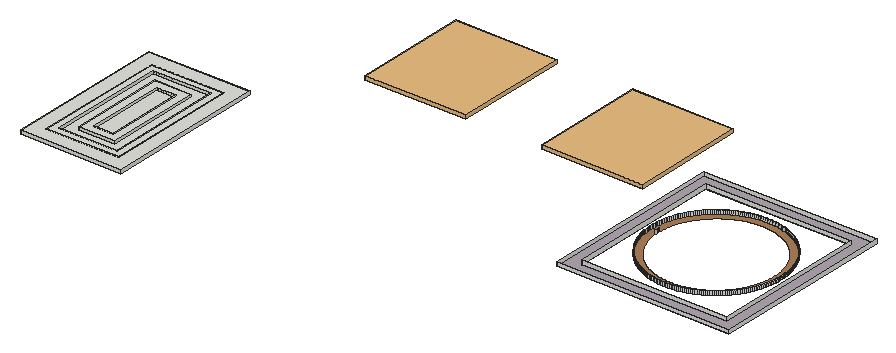
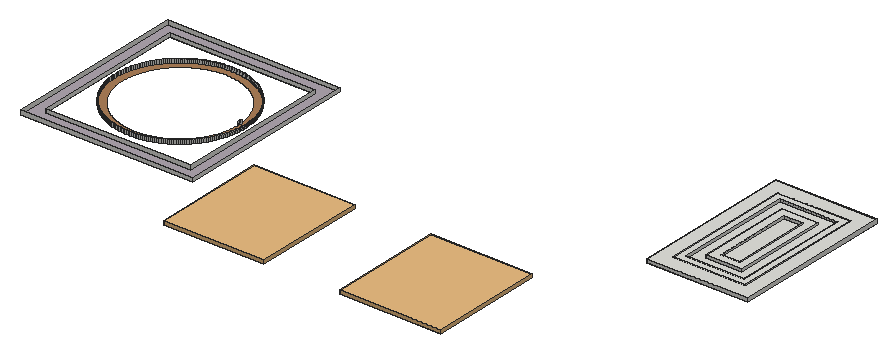
# SketchUp Ruby script. Lengths in inches.
U = 1.inch
M = Sketchup.active_model
def pt(a) = Geom::Point3d.new(a.map { |v| v * U })
def face(e, loops, mat)
  f = e.add_face(loops[0].map { |a| pt(a) })
  loops[1..].each { |l| e.add_face(l.map { |a| pt(a) }).erase! }
  f.material = f.back_material = mat if mat
  f
end
# faces: each face lists its corners as indices into pts; further lists are holes
def faces(e, pts, list, mat = nil) = list.each { |f| face(e, (f[0].is_a?(Array) ? f : [f]).map { |l| l.map { |i| pts[i] } }, mat) }
# xy, xz, yz: faces in a plane at the given z, y or x. An outline is a flat list of corners, or four numbers for a rectangle; further outlines are holes
def ring(l) = l.size == 4 ? [[l[0], l[1]], [l[2], l[1]], [l[2], l[3]], [l[0], l[3]]] : l.each_slice(2).to_a
def flat(e, list, mat, &to3) = list.each { |f| face(e, (f[0].is_a?(Array) ? f : [f]).map { |l| ring(l).map { |u, v| to3.(u, v) } }, mat) }
def xy(e, z, list, mat = nil) = flat(e, list, mat) { |x, y| [x, y, z] }
def xz(e, y, list, mat = nil) = flat(e, list, mat) { |x, z| [x, y, z] }
def yz(e, x, list, mat = nil) = flat(e, list, mat) { |y, z| [x, y, z] }
def lines(e, pts, list) = list.each { |a, b| e.add_line(pt(pts[a]), pt(pts[b])) }
# prism: a flat outline (further loops are holes) pulled along v
def prism(e, loops, v, mat = nil)
  f = face(e, loops, mat); d = Geom::Vector3d.new(v.map { |x| x * U })
  f.pushpull(f.normal.samedirection?(d) ? d.length : -d.length)
end
def box(e, o, s, mat = nil) = prism(e, [[o, [o[0] + s[0], o[1], o[2]], [o[0] + s[0], o[1] + s[1], o[2]], [o[0], o[1] + s[1], o[2]]]], [0, 0, s[2]], mat)
def at(x, y, z, deg = 0) = Geom::Transformation.translation(pt([x, y, z])) * Geom::Transformation.rotation(ORIGIN, Z_AXIS, deg.degrees)
def axes(o, x, y, z) = Geom::Transformation.new([*x, 0, *y, 0, *z, 0, *pt(o).to_a, 1])
def part(name) = M.definitions.add(name)
# library, detail: a bought-in or finely detailed component or shape, given as its bounding box
def library(name, o, s) = part(name).tap { |d| box(d.entities, o, s) }
def detail(e, o, s) = box(e.add_group.entities, o, s)
def put(e, d, t, mat = nil) = e.add_instance(d, t).tap { |i| i.material = mat if mat }
def group(e, t, mat = nil) = e.add_group.tap { |g| g.transformation = t; g.material = mat if mat }.entities
root = M.entities
M.materials.add("01 - Default1").color = [173, 128, 89]
M.materials.add("[0124_Purple]").color = [175, 166, 175]
c1 = library("Group\#54",[0,0,-6],[168,189,6])
c2 = library("Group\#57",[0,0,-6],[168,189,6])
xy(root,111,[[[761.98,172.26,1049.98,478.26],[785.98,196.26,1025.98,454.26]]],"[0124_Purple]")
xy(root,111.3125,[[[905.89,217.26,903.06,217.3,900.23,217.41,897.41,217.6,894.6,217.86,891.79,218.19,888.99,218.6,886.21,219.08,883.43,219.64,880.68,220.26,877.9375,220.96,875.22,221.73,872.52,222.57,869.84,223.48,867.1875,224.46,864.5625,225.51,861.97,226.63,859.4,227.82,856.86,229.07,854.36,230.39,851.9,231.77,849.47,233.22,847.08,234.73,844.73,236.3,842.42,237.9375,840.16,239.63,837.94,241.38,835.77,243.19,833.64,245.06,831.57,246.98,829.55,248.95,827.57,250.98,825.66,253.06,823.79,255.1875,821.99,257.36,820.24,259.58,818.55,261.85,816.92,264.16,815.35,266.51,813.84,268.91,812.4,271.34,811.02,273.81,809.71,276.31,808.46,278.85,807.28,281.41,806.16,284.01,805.12,286.64,804.14,289.29,803.24,291.97,802.4,294.67,801.63,297.39,800.94,300.13,800.32,302.89,799.77,305.67,799.29,308.45,798.89,311.25,798.5625,314.06,798.3,316.875,798.12,319.7,798.01,322.52,797.98,325.35,798.02,328.18,798.13,331,798.32,333.82,798.58,336.64,798.91,339.45,799.32,342.24,799.8,345.03,800.36,347.8,800.98,350.56,801.68,353.3,802.45,356.02,803.29,358.72,804.2,361.4,805.19,364.05,806.24,366.67,807.35,369.27,808.54,371.84,809.79,374.37,811.11,376.87,812.49,379.34,813.94,381.77,815.45,384.16,817.03,386.5,818.66,388.8125,820.35,391.08,822.11,393.3,823.92,395.47,825.78,397.59,827.7,399.67,829.68,401.69,831.7,403.66,833.78,405.58,835.91,407.44,838.08,409.25,840.31,411,842.57,412.68,844.88,414.31,847.24,415.88,849.63,417.39,852.06,418.83,854.53,420.21,857.03,421.53,859.57,422.78,862.14,423.96,864.74,425.07,867.36,426.12,870.02,427.09,872.69,428,875.39,428.84,878.12,429.6,880.86,430.29,883.62,430.92,886.39,431.46,889.18,431.94,891.97,432.34,894.78,432.67,897.6,432.93,900.42,433.11,903.24,433.22,906.07,433.26,908.9,433.22,911.72,433.1,914.55,432.92,917.36,432.65,920.17,432.32,922.97,431.91,925.75,431.43,928.52,430.875,931.28,430.25,934.02,429.55,936.74,428.78,939.44,427.94,942.12,427.03,944.77,426.05,947.39,425,949.99,423.88,952.56,422.7,955.09,421.44,957.59,420.125,960.06,418.74,962.49,417.29,964.88,415.78,967.23,414.21,969.53,412.58,971.8,410.88,974.02,409.13,976.19,407.32,978.3125,405.45,980.39,403.53,982.41,401.56,984.38,399.53,986.3,397.45,988.16,395.33,989.97,393.15,991.72,390.93,993.41,388.66,995.04,386.35,996.61,384,998.11,381.61,999.56,379.18,1000.94,376.71,1002.25,374.2,1003.5,371.67,1004.68,369.1,1005.79,366.5,1006.84,363.87,1007.82,361.22,1008.72,358.54,1009.56,355.84,1010.32,353.12,1011.02,350.38,1011.64,347.62,1012.1875,344.85,1012.66,342.06,1013.07,339.26,1013.4,336.45,1013.65,333.64,1013.84,330.82,1013.94,327.99,1013.98,325.16,1013.9375,322.34,1013.83,319.51,1013.64,316.69,1013.38,313.875,1013.04,311.07,1012.63,308.27,1012.15,305.48,1011.6,302.71,1010.97,299.95,1010.27,297.21,1009.5,294.49,1008.66,291.79,1007.75,289.12,1006.77,286.47,1005.72,283.84,1004.6,281.24,1003.42,278.68,1002.17,276.14,1000.85,273.64,999.46,271.18,998.02,268.75,996.5,266.36,994.93,264.01,993.3,261.7,991.6,259.4375,989.85,257.22,988.04,255.05,986.18,252.92,984.25,250.85,982.28,248.82,980.25,246.85,978.18,244.93,976.05,243.07,973.87,241.27,971.65,239.52,969.38,237.83,967.07,236.2,964.72,234.63,962.33,233.12,959.9,231.68,957.43,230.3,954.93,228.99,952.39,227.74,949.82,226.56,947.22,225.44,944.6,224.4,941.94,223.42,939.26,222.51,936.5625,221.68,933.84,220.91,931.1,220.22,928.34,219.6,925.57,219.05,922.78,218.57,919.98,218.17,917.18,217.84,914.36,217.58,911.54,217.4,908.71,217.29],[905.98,229.26,908.49,229.29,911,229.39,913.51,229.55,916.01,229.78,918.51,230.08,921,230.4375,923.47,230.86,925.9375,231.35,928.39,231.91,930.83,232.53,933.24,233.21,935.64,233.95,938.02,234.76,940.38,235.63,942.72,236.5625,945.03,237.56,947.31,238.61,949.5625,239.72,951.79,240.89,953.98,242.12,956.14,243.4,958.26,244.74,960.35,246.14,962.41,247.59,964.42,249.09,966.39,250.65,968.33,252.26,970.22,253.91,972.0625,255.62,973.86,257.375,975.61,259.17,977.32,261.02,978.98,262.91,980.58,264.84,982.14,266.82,983.64,268.83,985.09,270.88,986.49,272.97,987.83,275.1,989.12,277.26,990.35,279.45,991.52,281.67,992.625,283.93,993.68,286.21,994.67,288.52,995.6,290.85,996.47,293.21,997.28,295.59,998.03,297.99,998.71,300.41,999.33,302.85,999.88,305.3,1000.37,307.76,1000.8,310.24,1001.16,312.73,1001.45,315.22,1001.68,317.72,1001.85,320.23,1001.95,322.74,1001.98,325.26,1001.95,327.77,1001.85,330.28,1001.68,332.79,1001.45,335.29,1001.16,337.79,1000.8,340.27,1000.37,342.75,999.88,345.22,999.33,347.67,998.71,350.1,998.03,352.52,997.28,354.92,996.47,357.3,995.6,359.66,994.67,361.99,993.68,364.3,992.625,366.59,991.52,368.84,990.35,371.0625,989.12,373.26,987.83,375.42,986.49,377.54,985.09,379.63,983.64,381.68,982.14,383.7,980.58,385.67,978.98,387.6,977.32,389.49,975.61,391.34,973.86,393.14,972.0625,394.89,970.22,396.6,968.33,398.26,966.39,399.86,964.42,401.42,962.41,402.92,960.35,404.37,958.26,405.77,956.14,407.11,953.98,408.39,951.79,409.62,949.5625,410.79,947.31,411.9,945.03,412.96,942.72,413.95,940.38,414.88,938.02,415.75,935.64,416.56,933.24,417.3,930.83,417.99,928.39,418.6,925.9375,419.16,923.47,419.65,921,420.07,918.51,420.43,916.01,420.73,913.51,420.96,911,421.125,908.49,421.22,905.98,421.26,903.47,421.22,900.95,421.125,898.45,420.96,895.94,420.73,893.45,420.43,890.96,420.07,888.48,419.65,886.02,419.16,883.57,418.6,881.13,417.99,878.71,417.3,876.3125,416.56,873.93,415.75,871.58,414.88,869.24,413.95,866.93,412.96,864.65,411.9,862.4,410.79,860.17,409.62,857.98,408.39,855.82,407.11,853.69,405.77,851.6,404.37,849.55,402.92,847.54,401.42,845.5625,399.86,843.63,398.26,841.74,396.6,839.9,394.89,838.1,393.14,836.34,391.34,834.64,389.49,832.98,387.6,831.37,385.67,829.82,383.7,828.3125,381.68,826.86,379.63,825.47,377.54,824.125,375.42,822.84,373.26,821.61,371.0625,820.44,368.84,819.33,366.59,818.28,364.3,817.29,361.99,816.35,359.66,815.49,357.3,814.68,354.92,813.93,352.52,813.25,350.1,812.63,347.67,812.08,345.22,811.59,342.75,811.16,340.27,810.8,337.79,810.5,335.29,810.27,332.79,810.11,330.28,810.01,327.77,809.98,325.26,810.01,322.74,810.11,320.23,810.27,317.72,810.5,315.22,810.8,312.73,811.16,310.24,811.59,307.76,812.08,305.3,812.63,302.85,813.25,300.41,813.93,297.99,814.68,295.59,815.49,293.21,816.35,290.85,817.29,288.52,818.28,286.21,819.33,283.93,820.44,281.67,821.61,279.45,822.84,277.26,824.125,275.1,825.47,272.97,826.86,270.88,828.3125,268.83,829.82,266.82,831.37,264.84,832.98,262.91,834.64,261.02,836.34,259.17,838.1,257.375,839.9,255.62,841.74,253.91,843.63,252.26,845.5625,250.65,847.54,249.09,849.55,247.59,851.6,246.14,853.69,244.74,855.82,243.4,857.98,242.12,860.17,240.89,862.4,239.72,864.65,238.61,866.93,237.56,869.24,236.5625,871.58,235.63,873.93,234.76,876.3125,233.95,878.71,233.21,881.13,232.53,883.57,231.91,886.02,231.35,888.48,230.86,890.96,230.4375,893.45,230.08,895.94,229.78,898.45,229.55,900.95,229.39,903.47,229.29]]],"01 - Default1")
xz(root,172.26,[[761.98,111,1049.98,117.3125]])
xz(root,196.26,[[785.98,111,1025.98,117.3125]])
xz(root,454.26,[[785.98,111,1025.98,117.3125]])
xz(root,478.26,[[761.98,111,1049.98,117.3125]])
yz(root,761.98,[[172.26,111,478.26,117.3125]])
yz(root,785.98,[[196.26,111,454.26,117.3125]])
yz(root,1025.98,[[196.26,111,454.26,117.3125]])
yz(root,1049.98,[[172.26,111,478.26,117.3125]])
p = [[903.06,217.3,117.3125],[900.23,217.41,117.3125],[900.23,217.41,111.3125],[903.06,217.3,111.3125],[905.89,217.26,117.3125],[905.89,217.26,111.3125],
  [908.71,217.29,117.3125],[908.71,217.29,111.3125],[911.54,217.4,117.3125],[911.54,217.4,111.3125],[897.41,217.6,117.3125],[897.41,217.6,111.3125],
  [914.36,217.58,117.3125],[914.36,217.58,111.3125],[894.6,217.86,117.3125],[894.6,217.86,111.3125],[917.18,217.84,117.3125],[917.18,217.84,111.3125],
  [919.98,218.17,117.3125],[919.98,218.17,111.3125],[891.79,218.19,117.3125],[891.79,218.19,111.3125],[888.99,218.6,117.3125],[888.99,218.6,111.3125],
  [922.78,218.57,117.3125],[922.78,218.57,111.3125],[886.21,219.08,117.3125],[886.21,219.08,111.3125],[925.57,219.05,117.3125],[925.57,219.05,111.3125],
  [928.34,219.6,117.3125],[928.34,219.6,111.3125],[883.43,219.64,117.3125],[883.43,219.64,111.3125],[880.68,220.26,117.3125],[880.68,220.26,111.3125],
  [931.1,220.22,117.3125],[931.1,220.22,111.3125],[933.84,220.91,117.3125],[933.84,220.91,111.3125],[877.9375,220.96,117.3125],[877.9375,220.96,111.3125],
  [936.5625,221.68,117.3125],[936.5625,221.68,111.3125],[875.22,221.73,117.3125],[875.22,221.73,111.3125],[872.52,222.57,117.3125],[872.52,222.57,111.3125],
  [939.26,222.51,117.3125],[939.26,222.51,111.3125],[941.94,223.42,117.3125],[941.94,223.42,111.3125],[869.84,223.48,117.3125],[869.84,223.48,111.3125],
  [944.6,224.4,117.3125],[944.6,224.4,111.3125],[867.1875,224.46,117.3125],[867.1875,224.46,111.3125],[947.22,225.44,117.3125],[947.22,225.44,111.3125],
  [864.5625,225.51,117.3125],[864.5625,225.51,111.3125],[949.82,226.56,117.3125],[949.82,226.56,111.3125],[861.97,226.63,117.3125],[861.97,226.63,111.3125],
  [859.4,227.82,117.3125],[859.4,227.82,111.3125],[952.39,227.74,117.3125],[952.39,227.74,111.3125],[954.93,228.99,117.3125],[954.93,228.99,111.3125],
  [856.86,229.07,117.3125],[856.86,229.07,111.3125],[957.43,230.3,117.3125],[957.43,230.3,111.3125],[854.36,230.39,117.3125],[854.36,230.39,111.3125],
  [959.9,231.68,117.3125],[959.9,231.68,111.3125],[851.9,231.77,117.3125],[851.9,231.77,111.3125],[962.33,233.12,117.3125],[962.33,233.12,111.3125],
  [849.47,233.22,117.3125],[849.47,233.22,111.3125],[964.72,234.63,117.3125],[964.72,234.63,111.3125],[847.08,234.73,117.3125],[847.08,234.73,111.3125],
  [967.07,236.2,117.3125],[967.07,236.2,111.3125],[844.73,236.3,117.3125],[844.73,236.3,111.3125],[969.38,237.83,117.3125],[969.38,237.83,111.3125],
  [842.42,237.9375,117.3125],[842.42,237.9375,111.3125],[971.65,239.52,117.3125],[971.65,239.52,111.3125],[840.16,239.63,117.3125],[840.16,239.63,111.3125],
  [973.87,241.27,117.3125],[973.87,241.27,111.3125],[837.94,241.38,117.3125],[837.94,241.38,111.3125],[976.05,243.07,117.3125],[976.05,243.07,111.3125],
  [835.77,243.19,117.3125],[835.77,243.19,111.3125],[978.18,244.93,117.3125],[978.18,244.93,111.3125],[833.64,245.06,117.3125],[833.64,245.06,111.3125],
  [980.25,246.85,117.3125],[980.25,246.85,111.3125],[831.57,246.98,117.3125],[831.57,246.98,111.3125],[982.28,248.82,117.3125],[982.28,248.82,111.3125],
  [829.55,248.95,117.3125],[829.55,248.95,111.3125],[984.25,250.85,117.3125],[984.25,250.85,111.3125],[827.57,250.98,117.3125],[827.57,250.98,111.3125],
  [986.18,252.92,117.3125],[986.18,252.92,111.3125],[825.66,253.06,117.3125],[825.66,253.06,111.3125],[988.04,255.05,117.3125],[988.04,255.05,111.3125],
  [823.79,255.1875,117.3125],[823.79,255.1875,111.3125],[989.85,257.22,117.3125],[989.85,257.22,111.3125],[821.99,257.36,117.3125],[821.99,257.36,111.3125],
  [991.6,259.4375,117.3125],[991.6,259.4375,111.3125],[820.24,259.58,117.3125],[820.24,259.58,111.3125],[993.3,261.7,117.3125],[993.3,261.7,111.3125],
  [818.55,261.85,117.3125],[818.55,261.85,111.3125],[994.93,264.01,117.3125],[994.93,264.01,111.3125],[816.92,264.16,117.3125],[816.92,264.16,111.3125],
  [996.5,266.36,117.3125],[996.5,266.36,111.3125],[815.35,266.51,117.3125],[815.35,266.51,111.3125],[998.02,268.75,117.3125],[998.02,268.75,111.3125],
  [813.84,268.91,117.3125],[813.84,268.91,111.3125],[999.46,271.18,117.3125],[999.46,271.18,111.3125],[812.4,271.34,117.3125],[812.4,271.34,111.3125],
  [1000.85,273.64,117.3125],[1000.85,273.64,111.3125],[811.02,273.81,117.3125],[811.02,273.81,111.3125],[1002.17,276.14,117.3125],[1002.17,276.14,111.3125],
  [809.71,276.31,117.3125],[809.71,276.31,111.3125],[1003.42,278.68,117.3125],[1003.42,278.68,111.3125],[808.46,278.85,117.3125],[808.46,278.85,111.3125],
  [1004.6,281.24,117.3125],[1004.6,281.24,111.3125],[807.28,281.41,117.3125],[807.28,281.41,111.3125],[1005.72,283.84,117.3125],[1005.72,283.84,111.3125],
  [806.16,284.01,117.3125],[806.16,284.01,111.3125],[1006.77,286.47,117.3125],[1006.77,286.47,111.3125],[805.12,286.64,117.3125],[805.12,286.64,111.3125],
  [1007.75,289.12,117.3125],[1007.75,289.12,111.3125],[804.14,289.29,117.3125],[804.14,289.29,111.3125],[1008.66,291.79,117.3125],[1008.66,291.79,111.3125],
  [803.24,291.97,117.3125],[803.24,291.97,111.3125],[1009.5,294.49,117.3125],[1009.5,294.49,111.3125],[802.4,294.67,117.3125],[802.4,294.67,111.3125],
  [1010.27,297.21,117.3125],[1010.27,297.21,111.3125],[801.63,297.39,117.3125],[801.63,297.39,111.3125],[1010.97,299.95,117.3125],[1010.97,299.95,111.3125],
  [800.94,300.13,117.3125],[800.94,300.13,111.3125],[1011.6,302.71,117.3125],[1011.6,302.71,111.3125],[800.32,302.89,117.3125],[800.32,302.89,111.3125],
  [1012.15,305.48,117.3125],[1012.15,305.48,111.3125],[799.77,305.67,117.3125],[799.77,305.67,111.3125],[1012.63,308.27,117.3125],[1012.63,308.27,111.3125],
  [799.29,308.45,117.3125],[799.29,308.45,111.3125],[1013.04,311.07,117.3125],[1013.04,311.07,111.3125],[798.89,311.25,117.3125],[798.89,311.25,111.3125],
  [1013.38,313.875,117.3125],[1013.38,313.875,111.3125],[798.5625,314.06,117.3125],[798.5625,314.06,111.3125],[1013.64,316.69,117.3125],[1013.64,316.69,111.3125],
  [798.3,316.875,117.3125],[798.3,316.875,111.3125],[1013.83,319.51,117.3125],[1013.83,319.51,111.3125],[798.12,319.7,117.3125],[798.12,319.7,111.3125],
  [810.11,320.23,117.3125],[810.27,317.72,117.3125],[810.27,317.72,111.3125],[810.11,320.23,111.3125],[1013.9375,322.34,117.3125],[1013.9375,322.34,111.3125],
  [798.01,322.52,117.3125],[798.01,322.52,111.3125],[810.01,322.74,117.3125],[810.01,322.74,111.3125],[1013.98,325.16,117.3125],[1013.98,325.16,111.3125],
  [797.98,325.35,117.3125],[797.98,325.35,111.3125],[809.98,325.26,117.3125],[809.98,325.26,111.3125],[1013.94,327.99,117.3125],[1013.94,327.99,111.3125],
  [798.02,328.18,117.3125],[798.02,328.18,111.3125],[1013.84,330.82,117.3125],[1013.84,330.82,111.3125],[798.13,331,117.3125],[798.13,331,111.3125],
  [1013.65,333.64,117.3125],[1013.65,333.64,111.3125],[798.32,333.82,117.3125],[798.32,333.82,111.3125],[1013.4,336.45,117.3125],[1013.4,336.45,111.3125],
  [798.58,336.64,117.3125],[798.58,336.64,111.3125],[1013.07,339.26,117.3125],[1013.07,339.26,111.3125],[798.91,339.45,117.3125],[798.91,339.45,111.3125],
  [1012.66,342.06,117.3125],[1012.66,342.06,111.3125],[799.32,342.24,117.3125],[799.32,342.24,111.3125],[1012.1875,344.85,117.3125],[1012.1875,344.85,111.3125],
  [799.8,345.03,117.3125],[799.8,345.03,111.3125],[1011.64,347.62,117.3125],[1011.64,347.62,111.3125],[800.36,347.8,117.3125],[800.36,347.8,111.3125],
  [1011.02,350.38,117.3125],[1011.02,350.38,111.3125],[800.98,350.56,117.3125],[800.98,350.56,111.3125],[1010.32,353.12,117.3125],[1010.32,353.12,111.3125],
  [801.68,353.3,117.3125],[801.68,353.3,111.3125],[1009.56,355.84,117.3125],[1009.56,355.84,111.3125],[802.45,356.02,117.3125],[802.45,356.02,111.3125],
  [1008.72,358.54,117.3125],[1008.72,358.54,111.3125],[803.29,358.72,117.3125],[803.29,358.72,111.3125],[1007.82,361.22,117.3125],[1007.82,361.22,111.3125],
  [804.2,361.4,117.3125],[804.2,361.4,111.3125],[1006.84,363.87,117.3125],[1006.84,363.87,111.3125],[805.19,364.05,117.3125],[805.19,364.05,111.3125],
  [1005.79,366.5,117.3125],[1005.79,366.5,111.3125],[806.24,366.67,117.3125],[806.24,366.67,111.3125],[1004.68,369.1,117.3125],[1004.68,369.1,111.3125],
  [807.35,369.27,117.3125],[807.35,369.27,111.3125],[1003.5,371.67,117.3125],[1003.5,371.67,111.3125],[808.54,371.84,117.3125],[808.54,371.84,111.3125],
  [1002.25,374.2,117.3125],[1002.25,374.2,111.3125],[809.79,374.37,117.3125],[809.79,374.37,111.3125],[1000.94,376.71,117.3125],[1000.94,376.71,111.3125],
  [811.11,376.87,117.3125],[811.11,376.87,111.3125],[999.56,379.18,117.3125],[999.56,379.18,111.3125],[812.49,379.34,117.3125],[812.49,379.34,111.3125],
  [998.11,381.61,117.3125],[998.11,381.61,111.3125],[813.94,381.77,117.3125],[813.94,381.77,111.3125],[996.61,384,117.3125],[996.61,384,111.3125],
  [815.45,384.16,117.3125],[815.45,384.16,111.3125],[995.04,386.35,117.3125],[995.04,386.35,111.3125],[817.03,386.5,117.3125],[817.03,386.5,111.3125],
  [993.41,388.66,117.3125],[993.41,388.66,111.3125],[818.66,388.8125,117.3125],[818.66,388.8125,111.3125],[991.72,390.93,117.3125],[991.72,390.93,111.3125],
  [820.35,391.08,117.3125],[820.35,391.08,111.3125],[989.97,393.15,117.3125],[989.97,393.15,111.3125],[822.11,393.3,117.3125],[822.11,393.3,111.3125],
  [988.16,395.33,117.3125],[988.16,395.33,111.3125],[823.92,395.47,117.3125],[823.92,395.47,111.3125],[986.3,397.45,117.3125],[986.3,397.45,111.3125],
  [825.78,397.59,117.3125],[825.78,397.59,111.3125],[984.38,399.53,117.3125],[984.38,399.53,111.3125],[827.7,399.67,117.3125],[827.7,399.67,111.3125],
  [982.41,401.56,117.3125],[982.41,401.56,111.3125],[829.68,401.69,117.3125],[829.68,401.69,111.3125],[980.39,403.53,117.3125],[980.39,403.53,111.3125],
  [831.7,403.66,117.3125],[831.7,403.66,111.3125],[978.3125,405.45,117.3125],[978.3125,405.45,111.3125],[833.78,405.58,117.3125],[833.78,405.58,111.3125],
  [976.19,407.32,117.3125],[976.19,407.32,111.3125],[835.91,407.44,117.3125],[835.91,407.44,111.3125],[974.02,409.13,117.3125],[974.02,409.13,111.3125],
  [838.08,409.25,117.3125],[838.08,409.25,111.3125],[971.8,410.88,117.3125],[971.8,410.88,111.3125],[840.31,411,117.3125],[840.31,411,111.3125],
  [969.53,412.58,117.3125],[969.53,412.58,111.3125],[842.57,412.68,117.3125],[842.57,412.68,111.3125],[967.23,414.21,117.3125],[967.23,414.21,111.3125],
  [844.88,414.31,117.3125],[844.88,414.31,111.3125],[964.88,415.78,117.3125],[964.88,415.78,111.3125],[847.24,415.88,117.3125],[847.24,415.88,111.3125],
  [962.49,417.29,117.3125],[962.49,417.29,111.3125],[849.63,417.39,117.3125],[849.63,417.39,111.3125],[960.06,418.74,117.3125],[960.06,418.74,111.3125],
  [852.06,418.83,117.3125],[852.06,418.83,111.3125],[957.59,420.125,117.3125],[957.59,420.125,111.3125],[854.53,420.21,117.3125],[854.53,420.21,111.3125],
  [955.09,421.44,117.3125],[955.09,421.44,111.3125],[857.03,421.53,117.3125],[857.03,421.53,111.3125],[952.56,422.7,117.3125],[952.56,422.7,111.3125],
  [859.57,422.78,117.3125],[859.57,422.78,111.3125],[949.99,423.88,117.3125],[949.99,423.88,111.3125],[862.14,423.96,117.3125],[862.14,423.96,111.3125],
  [947.39,425,117.3125],[947.39,425,111.3125],[864.74,425.07,117.3125],[864.74,425.07,111.3125],[944.77,426.05,117.3125],[944.77,426.05,111.3125],
  [867.36,426.12,117.3125],[867.36,426.12,111.3125],[942.12,427.03,117.3125],[942.12,427.03,111.3125],[870.02,427.09,117.3125],[870.02,427.09,111.3125],
  [939.44,427.94,117.3125],[939.44,427.94,111.3125],[872.69,428,117.3125],[872.69,428,111.3125],[936.74,428.78,117.3125],[936.74,428.78,111.3125],
  [875.39,428.84,117.3125],[875.39,428.84,111.3125],[878.12,429.6,117.3125],[878.12,429.6,111.3125],[934.02,429.55,117.3125],[934.02,429.55,111.3125],
  [880.86,430.29,117.3125],[880.86,430.29,111.3125],[931.28,430.25,117.3125],[931.28,430.25,111.3125],[883.62,430.92,117.3125],[883.62,430.92,111.3125],
  [928.52,430.875,117.3125],[928.52,430.875,111.3125],[886.39,431.46,117.3125],[886.39,431.46,111.3125],[925.75,431.43,117.3125],[925.75,431.43,111.3125],
  [922.97,431.91,117.3125],[922.97,431.91,111.3125],[889.18,431.94,117.3125],[889.18,431.94,111.3125],[891.97,432.34,117.3125],[891.97,432.34,111.3125],
  [920.17,432.32,117.3125],[920.17,432.32,111.3125],[894.78,432.67,117.3125],[894.78,432.67,111.3125],[917.36,432.65,117.3125],[917.36,432.65,111.3125],
  [897.6,432.93,117.3125],[897.6,432.93,111.3125],[914.55,432.92,117.3125],[914.55,432.92,111.3125],[900.42,433.11,117.3125],[900.42,433.11,111.3125],
  [911.72,433.1,117.3125],[911.72,433.1,111.3125],[903.24,433.22,117.3125],[903.24,433.22,111.3125],[908.9,433.22,117.3125],[908.9,433.22,111.3125],
  [906.07,433.26,117.3125],[906.07,433.26,111.3125]]
faces(root,p,[[0,1,2,3],[4,0,3,5],[6,4,5,7],[8,6,7,9],[1,10,11,2],[12,8,9,13],[10,14,15,11],[16,12,13,17],
  [18,16,17,19],[14,20,21,15],[20,22,23,21],[24,18,19,25],[22,26,27,23],[28,24,25,29],[30,28,29,31],[26,32,33,27],
  [32,34,35,33],[36,30,31,37],[38,36,37,39],[34,40,41,35],[42,38,39,43],[40,44,45,41],[44,46,47,45],[48,42,43,49],
  [50,48,49,51],[46,52,53,47],[54,50,51,55],[52,56,57,53],[58,54,55,59],[56,60,61,57],[62,58,59,63],[60,64,65,61],
  [64,66,67,65],[68,62,63,69],[70,68,69,71],[66,72,73,67],[74,70,71,75],[72,76,77,73],[78,74,75,79],[76,80,81,77],
  [82,78,79,83],[80,84,85,81],[86,82,83,87],[84,88,89,85],[90,86,87,91],[88,92,93,89],[94,90,91,95],[92,96,97,93],
  [98,94,95,99],[96,100,101,97],[102,98,99,103],[100,104,105,101],[106,102,103,107],[104,108,109,105],[110,106,107,111],[108,112,113,109],
  [114,110,111,115],[112,116,117,113],[118,114,115,119],[116,120,121,117],[122,118,119,123],[120,124,125,121],[126,122,123,127],[124,128,129,125],
  [130,126,127,131],[128,132,133,129],[134,130,131,135],[132,136,137,133],[138,134,135,139],[136,140,141,137],[142,138,139,143],[140,144,145,141],
  [146,142,143,147],[144,148,149,145],[150,146,147,151],[148,152,153,149],[154,150,151,155],[152,156,157,153],[158,154,155,159],[156,160,161,157],
  [162,158,159,163],[160,164,165,161],[166,162,163,167],[164,168,169,165],[170,166,167,171],[168,172,173,169],[174,170,171,175],[172,176,177,173],
  [178,174,175,179],[176,180,181,177],[182,178,179,183],[180,184,185,181],[186,182,183,187],[184,188,189,185],[190,186,187,191],[188,192,193,189],
  [194,190,191,195],[192,196,197,193],[198,194,195,199],[196,200,201,197],[202,198,199,203],[200,204,205,201],[206,202,203,207],[204,208,209,205],
  [210,206,207,211],[208,212,213,209],[214,210,211,215],[212,216,217,213],[218,214,215,219],[216,220,221,217],[222,218,219,223],[220,224,225,221],
  [226,222,223,227],[224,228,229,225],[230,226,227,231],[228,232,233,229],[234,235,236,237],[238,230,231,239],[232,240,241,233],[242,234,237,243],
  [244,238,239,245],[240,246,247,241],[248,242,243,249],[250,244,245,251],[246,252,253,247],[254,250,251,255],[252,256,257,253],[258,254,255,259],
  [256,260,261,257],[262,258,259,263],[260,264,265,261],[266,262,263,267],[264,268,269,265],[270,266,267,271],[268,272,273,269],[274,270,271,275],
  [272,276,277,273],[278,274,275,279],[276,280,281,277],[282,278,279,283],[280,284,285,281],[286,282,283,287],[284,288,289,285],[290,286,287,291],
  [288,292,293,289],[294,290,291,295],[292,296,297,293],[298,294,295,299],[296,300,301,297],[302,298,299,303],[300,304,305,301],[306,302,303,307],
  [304,308,309,305],[310,306,307,311],[308,312,313,309],[314,310,311,315],[312,316,317,313],[318,314,315,319],[316,320,321,317],[322,318,319,323],
  [320,324,325,321],[326,322,323,327],[324,328,329,325],[330,326,327,331],[328,332,333,329],[334,330,331,335],[332,336,337,333],[338,334,335,339],
  [336,340,341,337],[342,338,339,343],[340,344,345,341],[346,342,343,347],[344,348,349,345],[350,346,347,351],[348,352,353,349],[354,350,351,355],
  [352,356,357,353],[358,354,355,359],[356,360,361,357],[362,358,359,363],[360,364,365,361],[366,362,363,367],[364,368,369,365],[370,366,367,371],
  [368,372,373,369],[374,370,371,375],[372,376,377,373],[378,374,375,379],[376,380,381,377],[382,378,379,383],[380,384,385,381],[386,382,383,387],
  [384,388,389,385],[390,386,387,391],[388,392,393,389],[394,390,391,395],[392,396,397,393],[398,394,395,399],[396,400,401,397],[402,398,399,403],
  [400,404,405,401],[406,402,403,407],[404,408,409,405],[410,406,407,411],[408,412,413,409],[414,410,411,415],[412,416,417,413],[418,414,415,419],
  [416,420,421,417],[422,418,419,423],[420,424,425,421],[426,422,423,427],[424,428,429,425],[430,426,427,431],[428,432,433,429],[434,430,431,435],
  [432,436,437,433],[438,434,435,439],[436,440,441,437],[442,438,439,443],[440,444,445,441],[444,446,447,445],[448,442,443,449],[446,450,451,447],
  [452,448,449,453],[450,454,455,451],[456,452,453,457],[454,458,459,455],[460,456,457,461],[462,460,461,463],[458,464,465,459],[464,466,467,465],
  [468,462,463,469],[466,470,471,467],[472,468,469,473],[470,474,475,471],[476,472,473,477],[474,478,479,475],[480,476,477,481],[478,482,483,479],
  [484,480,481,485],[482,486,487,483],[486,484,485,487]])
g1 = group(root,at(0,9,117.3125))
xy(g1,-6,[[[0,0,168,267],[24,24,144,243]]])
xy(g1,-4,[[[36,36,132,231],[54,54,114,213]],[67.77,67.77,100.23,199.23]])
xy(g1,0,[[[0,0,168,267],[24,24,144,243]],[[24,24,144,243],[36,36,132,231]],[[54,54,114,213],[67.77,67.77,100.23,199.23]]])
xz(g1,0,[[0,-6,168,0]])
xz(g1,24,[[24,-6,144,0]])
xz(g1,36,[[36,-4,132,0]])
xz(g1,54,[[54,-4,114,0]])
xz(g1,67.77,[[67.77,-4,100.23,0]])
xz(g1,199.23,[[67.77,-4,100.23,0]])
xz(g1,213,[[54,-4,114,0]])
xz(g1,231,[[36,-4,132,0]])
xz(g1,243,[[24,-6,144,0]])
xz(g1,267,[[0,-6,168,0]])
yz(g1,0,[[0,-6,267,0]])
yz(g1,24,[[24,-6,243,0]])
yz(g1,36,[[36,-4,231,0]])
yz(g1,54,[[54,-4,213,0]])
yz(g1,67.77,[[67.77,-4,199.23,0]])
yz(g1,100.23,[[67.77,-4,199.23,0]])
yz(g1,114,[[54,-4,213,0]])
yz(g1,132,[[36,-4,231,0]])
yz(g1,144,[[24,-6,243,0]])
yz(g1,168,[[0,-6,267,0]])
put(root,c1,at(553.625,402,117.3125))
put(root,c2,at(259.625,402,117.3125))
